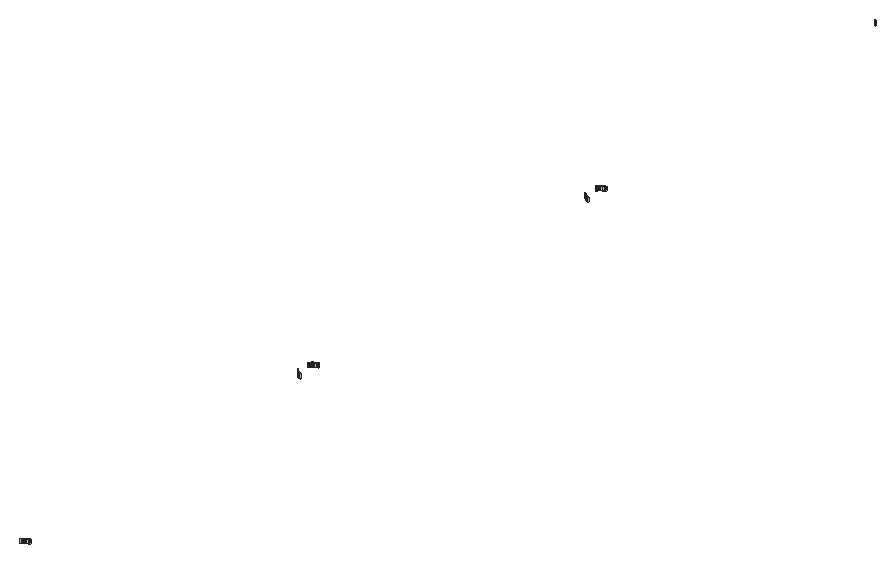
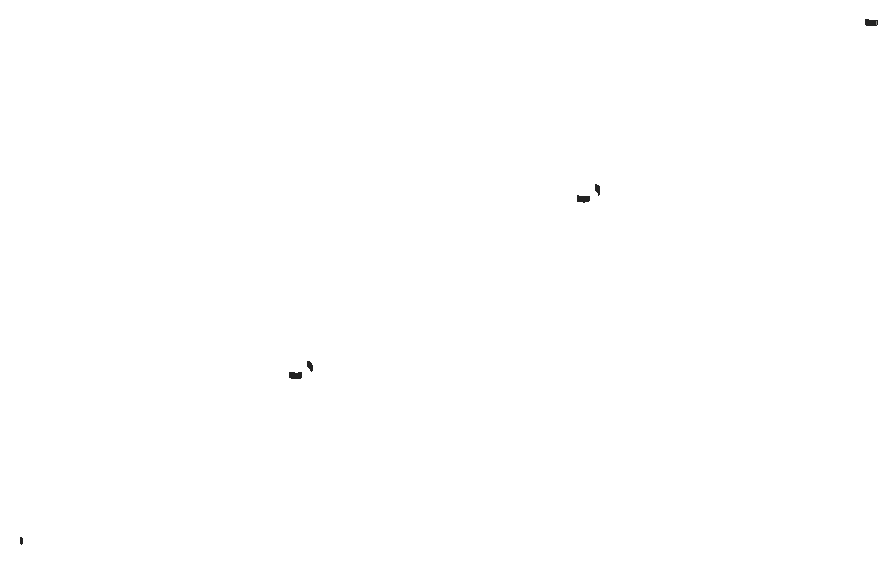
# SketchUp Ruby script. Lengths in inches.
U = 1.inch
M = Sketchup.active_model
def pt(a) = Geom::Point3d.new(a.map { |v| v * U })
def face(e, loops, mat)
  f = e.add_face(loops[0].map { |a| pt(a) })
  loops[1..].each { |l| e.add_face(l.map { |a| pt(a) }).erase! }
  f.material = f.back_material = mat if mat
  f
end
# faces: each face lists its corners as indices into pts; further lists are holes
def faces(e, pts, list, mat = nil) = list.each { |f| face(e, (f[0].is_a?(Array) ? f : [f]).map { |l| l.map { |i| pts[i] } }, mat) }
# xy, xz, yz: faces in a plane at the given z, y or x. An outline is a flat list of corners, or four numbers for a rectangle; further outlines are holes
def ring(l) = l.size == 4 ? [[l[0], l[1]], [l[2], l[1]], [l[2], l[3]], [l[0], l[3]]] : l.each_slice(2).to_a
def flat(e, list, mat, &to3) = list.each { |f| face(e, (f[0].is_a?(Array) ? f : [f]).map { |l| ring(l).map { |u, v| to3.(u, v) } }, mat) }
def xy(e, z, list, mat = nil) = flat(e, list, mat) { |x, y| [x, y, z] }
def xz(e, y, list, mat = nil) = flat(e, list, mat) { |x, z| [x, y, z] }
def yz(e, x, list, mat = nil) = flat(e, list, mat) { |y, z| [x, y, z] }
def lines(e, pts, list) = list.each { |a, b| e.add_line(pt(pts[a]), pt(pts[b])) }
# prism: a flat outline (further loops are holes) pulled along v
def prism(e, loops, v, mat = nil)
  f = face(e, loops, mat); d = Geom::Vector3d.new(v.map { |x| x * U })
  f.pushpull(f.normal.samedirection?(d) ? d.length : -d.length)
end
def box(e, o, s, mat = nil) = prism(e, [[o, [o[0] + s[0], o[1], o[2]], [o[0] + s[0], o[1] + s[1], o[2]], [o[0], o[1] + s[1], o[2]]]], [0, 0, s[2]], mat)
def at(x, y, z, deg = 0) = Geom::Transformation.translation(pt([x, y, z])) * Geom::Transformation.rotation(ORIGIN, Z_AXIS, deg.degrees)
def axes(o, x, y, z) = Geom::Transformation.new([*x, 0, *y, 0, *z, 0, *pt(o).to_a, 1])
def part(name) = M.definitions.add(name)
# library, detail: a bought-in or finely detailed component or shape, given as its bounding box
def library(name, o, s) = part(name).tap { |d| box(d.entities, o, s) }
def detail(e, o, s) = box(e.add_group.entities, o, s)
def put(e, d, t, mat = nil) = e.add_instance(d, t).tap { |i| i.material = mat if mat }
def group(e, t, mat = nil) = e.add_group.tap { |g| g.transformation = t; g.material = mat if mat }.entities
root = M.entities
p = [[357.57,250.76,128],[357.62,250.83,128],[357.62,250.83,129],[357.57,250.76,129],[357.67,250.89,128],[357.67,250.89,129],
  [357.72,250.95,128],[357.72,250.95,129],[357.77,251.01,128],[357.77,251.01,129],[357.82,251.07,128],[357.82,251.07,129],
  [357.88,251.12,128],[357.88,251.12,129],[357.93,251.18,128],[357.93,251.18,129],[357.99,251.23,128],[357.99,251.23,129],
  [358.05,251.28,128],[358.05,251.28,129],[358.11,251.33,128],[358.11,251.33,129],[358.17,251.38,128],[358.17,251.38,129],
  [358.24,251.43,128],[358.24,251.43,129],[358.3,251.47,128],[358.3,251.47,129],[358.37,251.52,128],[358.37,251.52,129],
  [358.43,251.56,128],[358.43,251.56,129],[358.5,251.6,128],[358.5,251.6,129],[358.57,251.64,128],[358.57,251.64,129],
  [358.64,251.67,128],[358.64,251.67,129],[358.71,251.71,128],[358.71,251.71,129],[358.78,251.74,128],[358.78,251.74,129],
  [358.85,251.77,128],[358.85,251.77,129],[358.92,251.8,128],[358.92,251.8,129],[359,251.83,128],[359,251.83,129],
  [359.07,251.85,128],[359.07,251.85,129],[359.15,251.875,128],[359.15,251.875,129],[359.22,251.9,128],[359.22,251.9,129],
  [359.3,251.92,128],[359.3,251.92,129],[359.375,251.93,128],[359.375,251.93,129],[359.07,339.15,128],[359,339.17,128],
  [359,339.17,129],[359.07,339.15,129],[359.15,339.125,128],[359.15,339.125,129],[359.22,339.1,128],[359.22,339.1,129],
  [359.3,339.08,128],[359.3,339.08,129],[358.85,339.23,128],[358.78,339.26,128],[358.78,339.26,129],[358.85,339.23,129],
  [358.92,339.2,128],[358.92,339.2,129],[358.64,339.33,128],[358.57,339.36,128],[358.57,339.36,129],[358.64,339.33,129],
  [358.71,339.29,128],[358.71,339.29,129],[358.43,339.44,128],[358.37,339.48,128],[358.37,339.48,129],[358.43,339.44,129],
  [358.5,339.4,128],[358.5,339.4,129],[358.3,339.53,128],[358.24,339.57,128],[358.24,339.57,129],[358.3,339.53,129],
  [358.17,339.62,128],[358.11,339.67,128],[358.11,339.67,129],[358.17,339.62,129],[358.05,339.72,128],[357.99,339.77,128],
  [357.99,339.77,129],[358.05,339.72,129],[357.93,339.82,128],[357.88,339.88,128],[357.88,339.88,129],[357.93,339.82,129],
  [357.82,339.93,128],[357.77,339.99,128],[357.77,339.99,129],[357.82,339.93,129],[357.72,340.05,128],[357.72,340.05,129],
  [357.67,340.11,128],[357.62,340.17,128],[357.62,340.17,129],[357.67,340.11,129],[357.57,340.24,128],[357.57,340.24,129],
  [357.53,343.7,128],[357.57,343.76,128],[357.57,343.76,129],[357.53,343.7,129],[357.62,343.83,128],[357.62,343.83,129],
  [357.67,343.89,128],[357.67,343.89,129],[357.72,343.95,128],[357.72,343.95,129],[357.77,344.01,128],[357.77,344.01,129],
  [357.82,344.07,128],[357.82,344.07,129],[357.88,344.12,128],[357.88,344.12,129],[357.93,344.18,128],[357.93,344.18,129],
  [357.99,344.23,128],[357.99,344.23,129],[358.05,344.28,128],[358.05,344.28,129],[358.11,344.33,128],[358.11,344.33,129],
  [358.17,344.38,128],[358.17,344.38,129],[358.24,344.43,128],[358.24,344.43,129],[358.3,344.47,128],[358.3,344.47,129],
  [358.37,344.52,128],[358.37,344.52,129],[358.43,344.56,128],[358.43,344.56,129],[358.5,344.6,128],[358.5,344.6,129],
  [358.57,344.64,128],[358.57,344.64,129],[358.64,344.67,128],[358.64,344.67,129],[358.71,344.71,128],[358.71,344.71,129],
  [358.78,344.74,128],[358.78,344.74,129],[358.85,344.77,128],[358.85,344.77,129],[358.92,344.8,128],[358.92,344.8,129],
  [359,344.83,128],[359,344.83,129],[359.07,344.85,128],[359.07,344.85,129],[359.15,344.875,128],[359.15,344.875,129],
  [359.22,344.9,128],[359.22,344.9,129],[359.3,344.92,128],[359.3,344.92,129],[359.375,344.93,128],[359.375,344.93,129],
  [359.07,432.15,128],[359,432.17,128],[359,432.17,129],[359.07,432.15,129],[359.15,432.125,128],[359.15,432.125,129],
  [359.22,432.1,128],[359.22,432.1,129],[359.3,432.08,128],[359.3,432.08,129],[358.85,432.23,128],[358.78,432.26,128],
  [358.78,432.26,129],[358.85,432.23,129],[358.92,432.2,128],[358.92,432.2,129],[358.64,432.33,128],[358.57,432.36,128],
  [358.57,432.36,129],[358.64,432.33,129],[358.71,432.29,128],[358.71,432.29,129],[358.43,432.44,128],[358.37,432.48,128],
  [358.37,432.48,129],[358.43,432.44,129],[358.5,432.4,128],[358.5,432.4,129],[358.3,432.53,128],[358.24,432.57,128],
  [358.24,432.57,129],[358.3,432.53,129],[358.17,432.62,128],[358.11,432.67,128],[358.11,432.67,129],[358.17,432.62,129],
  [358.05,432.72,128],[357.99,432.77,128],[357.99,432.77,129],[358.05,432.72,129],[357.93,432.82,128],[357.88,432.88,128],
  [357.88,432.88,129],[357.93,432.82,129],[357.82,432.93,128],[357.77,432.99,128],[357.77,432.99,129],[357.82,432.93,129],
  [357.72,433.05,128],[357.72,433.05,129],[357.67,433.11,128],[357.62,433.17,128],[357.62,433.17,129],[357.67,433.11,129],
  [357.57,433.24,128],[357.53,433.3,128],[357.53,433.3,129],[357.57,433.24,129],[357.53,436.7,128],[357.57,436.76,128],
  [357.57,436.76,129],[357.53,436.7,129],[357.62,436.83,128],[357.62,436.83,129],[357.67,436.89,128],[357.67,436.89,129],
  [357.72,436.95,128],[357.72,436.95,129],[357.77,437.01,128],[357.77,437.01,129],[357.82,437.07,128],[357.82,437.07,129],
  [357.88,437.12,128],[357.88,437.12,129],[357.93,437.18,128],[357.93,437.18,129],[357.99,437.23,128],[357.99,437.23,129],
  [358.05,437.28,128],[358.05,437.28,129],[358.11,437.33,128],[358.11,437.33,129],[358.17,437.38,128],[358.17,437.38,129],
  [358.24,437.43,128],[358.24,437.43,129],[358.3,437.47,128],[358.3,437.47,129],[358.37,437.52,128],[358.37,437.52,129],
  [358.43,437.56,128],[358.43,437.56,129],[358.5,437.6,128],[358.5,437.6,129],[358.57,437.64,128],[358.57,437.64,129],
  [358.64,437.67,128],[358.64,437.67,129],[358.71,437.71,128],[358.71,437.71,129],[358.78,437.74,128],[358.78,437.74,129],
  [358.85,437.77,128],[358.85,437.77,129],[358.92,437.8,128],[358.92,437.8,129],[359,437.83,128],[359,437.83,129],
  [359.07,437.85,128],[359.07,437.85,129],[359.15,437.875,128],[359.15,437.875,129],[359.22,437.9,128],[359.22,437.9,129],
  [359.3,437.92,128],[359.3,437.92,129],[359.07,525.15,128],[359,525.17,128],[359,525.17,129],[359.07,525.15,129],
  [359.15,525.125,128],[359.15,525.125,129],[359.22,525.1,128],[359.22,525.1,129],[359.3,525.08,128],[359.3,525.08,129],
  [358.85,525.23,128],[358.78,525.26,128],[358.78,525.26,129],[358.85,525.23,129],[358.92,525.2,128],[358.92,525.2,129],
  [358.71,525.29,128],[358.64,525.33,128],[358.64,525.33,129],[358.71,525.29,129]]
faces(root,p,[[0,1,2,3],[1,4,5,2],[4,6,7,5],[6,8,9,7],[8,10,11,9],[10,12,13,11],[12,14,15,13],[14,16,17,15],
  [16,18,19,17],[18,20,21,19],[20,22,23,21],[22,24,25,23],[24,26,27,25],[26,28,29,27],[28,30,31,29],[30,32,33,31],
  [32,34,35,33],[34,36,37,35],[36,38,39,37],[38,40,41,39],[40,42,43,41],[42,44,45,43],[44,46,47,45],[46,48,49,47],
  [48,50,51,49],[50,52,53,51],[52,54,55,53],[54,56,57,55],[58,59,60,61],[62,58,61,63],[64,62,63,65],[66,64,65,67],
  [68,69,70,71],[72,68,71,73],[59,72,73,60],[74,75,76,77],[78,74,77,79],[69,78,79,70],[80,81,82,83],[84,80,83,85],
  [75,84,85,76],[86,87,88,89],[81,86,89,82],[90,91,92,93],[87,90,93,88],[94,95,96,97],[91,94,97,92],[98,99,100,101],
  [95,98,101,96],[102,103,104,105],[99,102,105,100],[103,106,107,104],[108,109,110,111],[106,108,111,107],[109,112,113,110],[114,115,116,117],
  [115,118,119,116],[118,120,121,119],[120,122,123,121],[122,124,125,123],[124,126,127,125],[126,128,129,127],[128,130,131,129],[130,132,133,131],
  [132,134,135,133],[134,136,137,135],[136,138,139,137],[138,140,141,139],[140,142,143,141],[142,144,145,143],[144,146,147,145],[146,148,149,147],
  [148,150,151,149],[150,152,153,151],[152,154,155,153],[154,156,157,155],[156,158,159,157],[158,160,161,159],[160,162,163,161],[162,164,165,163],
  [164,166,167,165],[166,168,169,167],[168,170,171,169],[170,172,173,171],[174,175,176,177],[178,174,177,179],[180,178,179,181],[182,180,181,183],
  [184,185,186,187],[188,184,187,189],[175,188,189,176],[190,191,192,193],[194,190,193,195],[185,194,195,186],[196,197,198,199],[200,196,199,201],
  [191,200,201,192],[202,203,204,205],[197,202,205,198],[206,207,208,209],[203,206,209,204],[210,211,212,213],[207,210,213,208],[214,215,216,217],
  [211,214,217,212],[218,219,220,221],[215,218,221,216],[219,222,223,220],[224,225,226,227],[222,224,227,223],[228,229,230,231],[225,228,231,226],
  [232,233,234,235],[233,236,237,234],[236,238,239,237],[238,240,241,239],[240,242,243,241],[242,244,245,243],[244,246,247,245],[246,248,249,247],
  [248,250,251,249],[250,252,253,251],[252,254,255,253],[254,256,257,255],[256,258,259,257],[258,260,261,259],[260,262,263,261],[262,264,265,263],
  [264,266,267,265],[266,268,269,267],[268,270,271,269],[270,272,273,271],[272,274,275,273],[274,276,277,275],[276,278,279,277],[278,280,281,279],
  [280,282,283,281],[282,284,285,283],[284,286,287,285],[286,288,289,287],[290,291,292,293],[294,290,293,295],[296,294,295,297],[298,296,297,299],
  [300,301,302,303],[304,300,303,305],[291,304,305,292],[306,307,308,309],[301,306,309,302]])
